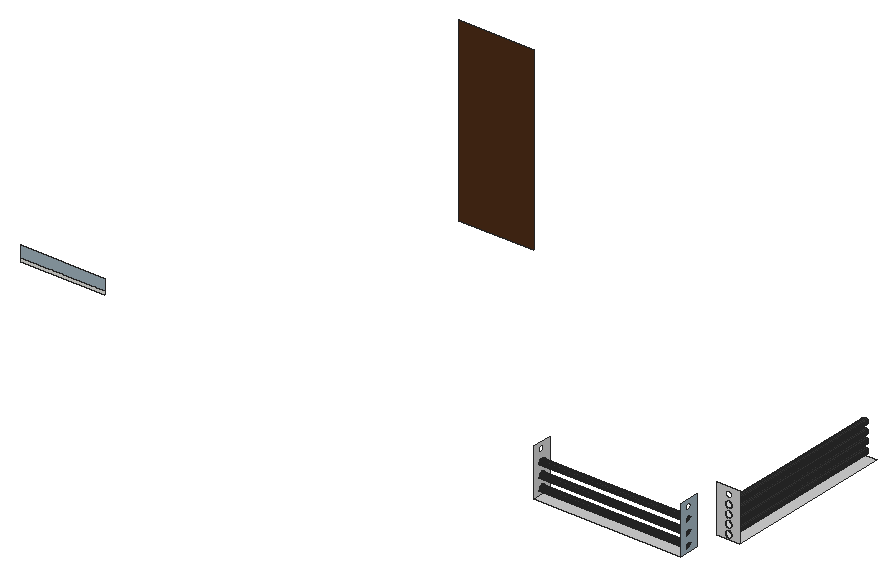
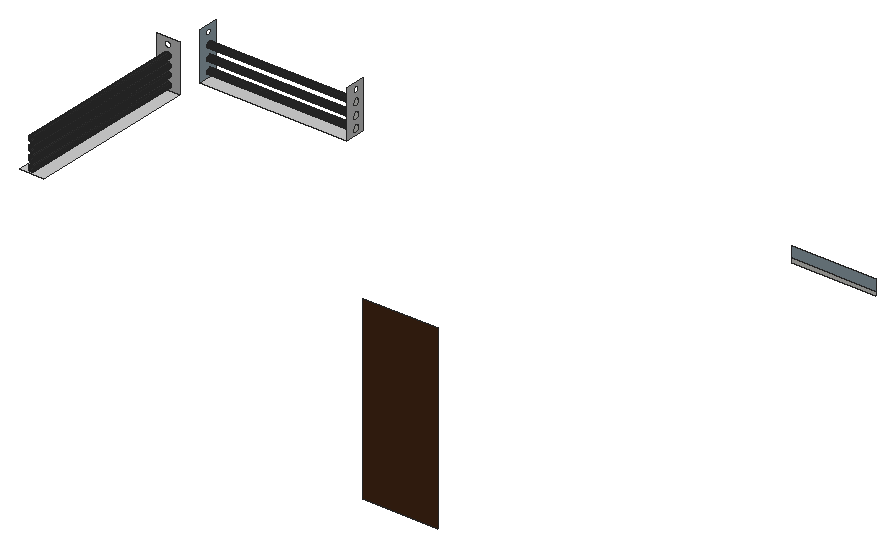
# SketchUp Ruby script. Lengths in inches.
U = 1.inch
M = Sketchup.active_model
def pt(a) = Geom::Point3d.new(a.map { |v| v * U })
def face(e, loops, mat)
  f = e.add_face(loops[0].map { |a| pt(a) })
  loops[1..].each { |l| e.add_face(l.map { |a| pt(a) }).erase! }
  f.material = f.back_material = mat if mat
  f
end
# faces: each face lists its corners as indices into pts; further lists are holes
def faces(e, pts, list, mat = nil) = list.each { |f| face(e, (f[0].is_a?(Array) ? f : [f]).map { |l| l.map { |i| pts[i] } }, mat) }
# xy, xz, yz: faces in a plane at the given z, y or x. An outline is a flat list of corners, or four numbers for a rectangle; further outlines are holes
def ring(l) = l.size == 4 ? [[l[0], l[1]], [l[2], l[1]], [l[2], l[3]], [l[0], l[3]]] : l.each_slice(2).to_a
def flat(e, list, mat, &to3) = list.each { |f| face(e, (f[0].is_a?(Array) ? f : [f]).map { |l| ring(l).map { |u, v| to3.(u, v) } }, mat) }
def xy(e, z, list, mat = nil) = flat(e, list, mat) { |x, y| [x, y, z] }
def xz(e, y, list, mat = nil) = flat(e, list, mat) { |x, z| [x, y, z] }
def yz(e, x, list, mat = nil) = flat(e, list, mat) { |y, z| [x, y, z] }
def lines(e, pts, list) = list.each { |a, b| e.add_line(pt(pts[a]), pt(pts[b])) }
# prism: a flat outline (further loops are holes) pulled along v
def prism(e, loops, v, mat = nil)
  f = face(e, loops, mat); d = Geom::Vector3d.new(v.map { |x| x * U })
  f.pushpull(f.normal.samedirection?(d) ? d.length : -d.length)
end
def box(e, o, s, mat = nil) = prism(e, [[o, [o[0] + s[0], o[1], o[2]], [o[0] + s[0], o[1] + s[1], o[2]], [o[0], o[1] + s[1], o[2]]]], [0, 0, s[2]], mat)
def at(x, y, z, deg = 0) = Geom::Transformation.translation(pt([x, y, z])) * Geom::Transformation.rotation(ORIGIN, Z_AXIS, deg.degrees)
def axes(o, x, y, z) = Geom::Transformation.new([*x, 0, *y, 0, *z, 0, *pt(o).to_a, 1])
def part(name) = M.definitions.add(name)
# library, detail: a bought-in or finely detailed component or shape, given as its bounding box
def library(name, o, s) = part(name).tap { |d| box(d.entities, o, s) }
def detail(e, o, s) = box(e.add_group.entities, o, s)
def put(e, d, t, mat = nil) = e.add_instance(d, t).tap { |i| i.material = mat if mat }
def group(e, t, mat = nil) = e.add_group.tap { |g| g.transformation = t; g.material = mat if mat }.entities
root = M.entities
M.materials.add("[Carrera Marble]").color = [207, 207, 207]
M.materials.add("[Color M07]").color = [58, 58, 58]
M.materials.add("[Formica Speckled Grey]").color = [157, 176, 186]
M.materials.add("[Quartz Light Grey]").color = [251, 251, 252]
M.materials.add("[Wood Veneer 01]").color = [76, 44, 23]
xy(root,72.8125,[[580.71,195.25,736.96,216.53],[736.96,242.62,761.74,423.625]],"[Carrera Marble]")
xz(root,195.25,[[36.42,107.15,126.39,111.12]])
xz(root,195.25,[[36.42,111.12,126.39,122.8125]],"[Formica Speckled Grey]")
xz(root,242.62,[[[736.96,72.8125,761.74,122.8125],[749.95,112.77,749.11,112.88,748.32,113.2,747.65,113.72,747.13,114.39,746.81,115.18,746.7,116.02,746.81,116.86,747.13,117.64,747.65,118.32,748.32,118.83,749.11,119.16,749.95,119.27,750.79,119.16,751.57,118.83,752.24,118.32,752.76,117.64,753.09,116.86,753.2,116.02,753.09,115.18,752.76,114.39,752.24,113.72,751.57,113.2,750.79,112.88],[749.95,74.64,749.11,74.75,748.32,75.08,747.65,75.59,747.13,76.27,746.81,77.05,746.7,77.89,746.81,78.73,747.13,79.52,747.65,80.19,748.32,80.71,749.11,81.03,749.95,81.14,750.79,81.03,751.57,80.71,752.24,80.19,752.76,79.52,753.09,78.73,753.2,77.89,753.09,77.05,752.76,76.27,752.24,75.59,751.57,75.08,750.79,74.75],[749.95,102.77,749.11,102.88,748.32,103.2,747.65,103.72,747.13,104.39,746.81,105.18,746.7,106.02,746.81,106.86,747.13,107.64,747.65,108.32,748.32,108.83,749.11,109.16,749.95,109.27,750.79,109.16,751.57,108.83,752.24,108.32,752.76,107.64,753.09,106.86,753.2,106.02,753.09,105.18,752.76,104.39,752.24,103.72,751.57,103.2,750.79,102.88],[749.95,84.2,749.11,84.32,748.32,84.64,747.65,85.16,747.13,85.83,746.81,86.61,746.7,87.45,746.81,88.3,747.13,89.08,747.65,89.75,748.32,90.27,749.11,90.59,749.95,90.7,750.79,90.59,751.57,90.27,752.24,89.75,752.76,89.08,753.09,88.3,753.2,87.45,753.09,86.61,752.76,85.83,752.24,85.16,751.57,84.64,750.79,84.32],[749.95,93.33,749.11,93.44,748.32,93.77,747.65,94.28,747.13,94.95,746.81,95.74,746.7,96.58,746.81,97.42,747.13,98.2,747.65,98.88,748.32,99.39,749.11,99.72,749.95,99.83,750.79,99.72,751.57,99.39,752.24,98.88,752.76,98.2,753.09,97.42,753.2,96.58,753.09,95.74,752.76,94.95,752.24,94.28,751.57,93.77,750.79,93.44]]],"[Carrera Marble]")
xz(root,242.62,[[749.95,74.64,750.79,74.75,751.57,75.08,752.24,75.59,752.76,76.27,753.09,77.05,753.2,77.89,753.09,78.73,752.76,79.52,752.24,80.19,751.57,80.71,750.79,81.03,749.95,81.14,749.11,81.03,748.32,80.71,747.65,80.19,747.13,79.52,746.81,78.73,746.7,77.89,746.81,77.05,747.13,76.27,747.65,75.59,748.32,75.08,749.11,74.75],[749.95,84.2,750.79,84.32,751.57,84.64,752.24,85.16,752.76,85.83,753.09,86.61,753.2,87.45,753.09,88.3,752.76,89.08,752.24,89.75,751.57,90.27,750.79,90.59,749.95,90.7,749.11,90.59,748.32,90.27,747.65,89.75,747.13,89.08,746.81,88.3,746.7,87.45,746.81,86.61,747.13,85.83,747.65,85.16,748.32,84.64,749.11,84.32],[749.95,93.33,750.79,93.44,751.57,93.77,752.24,94.28,752.76,94.95,753.09,95.74,753.2,96.58,753.09,97.42,752.76,98.2,752.24,98.88,751.57,99.39,750.79,99.72,749.95,99.83,749.11,99.72,748.32,99.39,747.65,98.88,747.13,98.2,746.81,97.42,746.7,96.58,746.81,95.74,747.13,94.95,747.65,94.28,748.32,93.77,749.11,93.44],[749.95,102.77,750.79,102.88,751.57,103.2,752.24,103.72,752.76,104.39,753.09,105.18,753.2,106.02,753.09,106.86,752.76,107.64,752.24,108.32,751.57,108.83,750.79,109.16,749.95,109.27,749.11,109.16,748.32,108.83,747.65,108.32,747.13,107.64,746.81,106.86,746.7,106.02,746.81,105.18,747.13,104.39,747.65,103.72,748.32,103.2,749.11,102.88]],"[Quartz Light Grey]")
xz(root,602.92,[[175.34,16.18,255.42,206.57]],"[Wood Veneer 01]")
yz(root,580.71,[[205.03,76.17,204.24,76.27,203.5,76.58,202.87,77.06,202.38,77.7,202.08,78.4375,201.97,79.23,202.08,80.02,202.38,80.76,202.87,81.4,203.5,81.88,204.24,82.1875,205.03,82.29,205.83,82.1875,206.57,81.88,207.2,81.4,207.6875,80.76,207.99,80.02,208.1,79.23,207.99,78.4375,207.6875,77.7,207.2,77.06,206.57,76.58,205.83,76.27],[205.03,88.54,204.24,88.65,203.5,88.95,202.87,89.44,202.38,90.07,202.08,90.8125,201.97,91.61,202.08,92.4,202.38,93.14,202.87,93.77,203.5,94.26,204.24,94.5625,205.03,94.67,205.83,94.5625,206.57,94.26,207.2,93.77,207.6875,93.14,207.99,92.4,208.1,91.61,207.99,90.8125,207.6875,90.07,207.2,89.44,206.57,88.95,205.83,88.65],[205.03,101.48,204.24,101.58,203.5,101.89,202.87,102.38,202.38,103.01,202.08,103.75,201.97,104.54,202.08,105.34,202.38,106.07,202.87,106.71,203.5,107.2,204.24,107.5,205.03,107.61,205.83,107.5,206.57,107.2,207.2,106.71,207.6875,106.07,207.99,105.34,208.1,104.54,207.99,103.75,207.6875,103.01,207.2,102.38,206.57,101.89,205.83,101.58]])
yz(root,580.71,[[[195.25,72.8125,216.53,122.8125],[205.03,76.17,204.24,76.27,203.5,76.58,202.87,77.06,202.38,77.7,202.08,78.4375,201.97,79.23,202.08,80.02,202.38,80.76,202.87,81.4,203.5,81.88,204.24,82.1875,205.03,82.29,205.83,82.1875,206.57,81.88,207.2,81.4,207.6875,80.76,207.99,80.02,208.1,79.23,207.99,78.4375,207.6875,77.7,207.2,77.06,206.57,76.58,205.83,76.27],[205.03,101.48,204.24,101.58,203.5,101.89,202.87,102.38,202.38,103.01,202.08,103.75,201.97,104.54,202.08,105.34,202.38,106.07,202.87,106.71,203.5,107.2,204.24,107.5,205.03,107.61,205.83,107.5,206.57,107.2,207.2,106.71,207.6875,106.07,207.99,105.34,208.1,104.54,207.99,103.75,207.6875,103.01,207.2,102.38,206.57,101.89,205.83,101.58],[205.03,88.54,204.24,88.65,203.5,88.95,202.87,89.44,202.38,90.07,202.08,90.8125,201.97,91.61,202.08,92.4,202.38,93.14,202.87,93.77,203.5,94.26,204.24,94.5625,205.03,94.67,205.83,94.5625,206.57,94.26,207.2,93.77,207.6875,93.14,207.99,92.4,208.1,91.61,207.99,90.8125,207.6875,90.07,207.2,89.44,206.57,88.95,205.83,88.65],[205.03,113.17,204.24,113.27,203.5,113.58,202.87,114.06,202.38,114.7,202.08,115.4375,201.97,116.23,202.08,117.02,202.38,117.76,202.87,118.4,203.5,118.88,204.24,119.1875,205.03,119.29,205.83,119.1875,206.57,118.88,207.2,118.4,207.6875,117.76,207.99,117.02,208.1,116.23,207.99,115.4375,207.6875,114.7,207.2,114.06,206.57,113.58,205.83,113.27]]],"[Carrera Marble]")
yz(root,736.96,[[[195.25,72.8125,216.53,122.8125],[205.03,113.17,204.24,113.27,203.5,113.58,202.87,114.06,202.38,114.7,202.08,115.4375,201.97,116.23,202.08,117.02,202.38,117.76,202.87,118.4,203.5,118.88,204.24,119.1875,205.03,119.29,205.83,119.1875,206.57,118.88,207.2,118.4,207.6875,117.76,207.99,117.02,208.1,116.23,207.99,115.4375,207.6875,114.7,207.2,114.06,206.57,113.58,205.83,113.27],[205.03,101.48,204.24,101.58,203.5,101.89,202.87,102.38,202.38,103.01,202.08,103.75,201.97,104.54,202.08,105.34,202.38,106.07,202.87,106.71,203.5,107.2,204.24,107.5,205.03,107.61,205.83,107.5,206.57,107.2,207.2,106.71,207.6875,106.07,207.99,105.34,208.1,104.54,207.99,103.75,207.6875,103.01,207.2,102.38,206.57,101.89,205.83,101.58],[205.03,88.54,204.24,88.65,203.5,88.95,202.87,89.44,202.38,90.07,202.08,90.8125,201.97,91.61,202.08,92.4,202.38,93.14,202.87,93.77,203.5,94.26,204.24,94.5625,205.03,94.67,205.83,94.5625,206.57,94.26,207.2,93.77,207.6875,93.14,207.99,92.4,208.1,91.61,207.99,90.8125,207.6875,90.07,207.2,89.44,206.57,88.95,205.83,88.65],[205.03,76.17,204.24,76.27,203.5,76.58,202.87,77.06,202.38,77.7,202.08,78.4375,201.97,79.23,202.08,80.02,202.38,80.76,202.87,81.4,203.5,81.88,204.24,82.1875,205.03,82.29,205.83,82.1875,206.57,81.88,207.2,81.4,207.6875,80.76,207.99,80.02,208.1,79.23,207.99,78.4375,207.6875,77.7,207.2,77.06,206.57,76.58,205.83,76.27]]],"[Formica Speckled Grey]")
p = [[749.95,242.62,74.64],[749.11,242.62,74.75],[749.11,423.625,74.75],[749.95,423.625,74.64],[750.79,242.62,74.75],[750.79,423.625,74.75],
  [748.32,242.62,75.08],[748.32,423.625,75.08],[751.57,242.62,75.08],[751.57,423.625,75.08],[747.65,242.62,75.59],[747.65,423.625,75.59],
  [752.24,242.62,75.59],[752.24,423.625,75.59],[747.13,242.62,76.27],[747.13,423.625,76.27],[752.76,242.62,76.27],[752.76,423.625,76.27],
  [580.71,204.24,76.27],[580.71,205.03,76.17],[736.96,205.03,76.17],[736.96,204.24,76.27],[580.71,205.83,76.27],[736.96,205.83,76.27],
  [580.71,203.5,76.58],[736.96,203.5,76.58],[580.71,206.57,76.58],[736.96,206.57,76.58],[746.81,242.62,77.05],[746.81,423.625,77.05],
  [753.09,242.62,77.05],[753.09,423.625,77.05],[580.71,202.87,77.06],[736.96,202.87,77.06],[580.71,207.2,77.06],[736.96,207.2,77.06],
  [580.71,202.38,77.7],[736.96,202.38,77.7],[580.71,207.6875,77.7],[736.96,207.6875,77.7],[746.7,242.62,77.89],[746.7,423.625,77.89],
  [753.2,242.62,77.89],[753.2,423.625,77.89],[580.71,202.08,78.4375],[736.96,202.08,78.4375],[580.71,207.99,78.4375],[736.96,207.99,78.4375],
  [746.81,242.62,78.73],[746.81,423.625,78.73],[753.09,242.62,78.73],[753.09,423.625,78.73],[580.71,201.97,79.23],[736.96,201.97,79.23],
  [580.71,208.1,79.23],[736.96,208.1,79.23],[747.13,242.62,79.52],[747.13,423.625,79.52],[752.76,242.62,79.52],[752.76,423.625,79.52],
  [580.71,202.08,80.02],[736.96,202.08,80.02],[580.71,207.99,80.02],[736.96,207.99,80.02],[747.65,242.62,80.19],[747.65,423.625,80.19],
  [752.24,242.62,80.19],[752.24,423.625,80.19],[580.71,202.38,80.76],[736.96,202.38,80.76],[580.71,207.6875,80.76],[736.96,207.6875,80.76],
  [748.32,242.62,80.71],[748.32,423.625,80.71],[751.57,242.62,80.71],[751.57,423.625,80.71],[749.11,242.62,81.03],[749.11,423.625,81.03],
  [750.79,242.62,81.03],[750.79,423.625,81.03],[580.71,202.87,81.4],[736.96,202.87,81.4],[580.71,207.2,81.4],[736.96,207.2,81.4],
  [749.95,242.62,81.14],[749.95,423.625,81.14],[580.71,203.5,81.88],[736.96,203.5,81.88],[580.71,206.57,81.88],[736.96,206.57,81.88],
  [580.71,204.24,82.1875],[736.96,204.24,82.1875],[580.71,205.83,82.1875],[736.96,205.83,82.1875],[580.71,205.03,82.29],[736.96,205.03,82.29],
  [749.95,242.62,84.2],[749.11,242.62,84.32],[749.11,423.625,84.32],[749.95,423.625,84.2],[750.79,242.62,84.32],[750.79,423.625,84.32],
  [748.32,242.62,84.64],[748.32,423.625,84.64],[751.57,242.62,84.64],[751.57,423.625,84.64],[747.65,242.62,85.16],[747.65,423.625,85.16],
  [752.24,242.62,85.16],[752.24,423.625,85.16],[747.13,242.62,85.83],[747.13,423.625,85.83],[752.76,242.62,85.83],[752.76,423.625,85.83],
  [746.81,242.62,86.61],[746.81,423.625,86.61],[753.09,242.62,86.61],[753.09,423.625,86.61],[746.7,242.62,87.45],[746.7,423.625,87.45],
  [753.2,242.62,87.45],[753.2,423.625,87.45],[746.81,242.62,88.3],[746.81,423.625,88.3],[753.09,242.62,88.3],[753.09,423.625,88.3],
  [747.13,242.62,89.08],[747.13,423.625,89.08],[752.76,242.62,89.08],[752.76,423.625,89.08],[580.71,204.24,88.65],[580.71,205.03,88.54],
  [736.96,205.03,88.54],[736.96,204.24,88.65],[580.71,205.83,88.65],[736.96,205.83,88.65],[580.71,203.5,88.95],[736.96,203.5,88.95],
  [580.71,206.57,88.95],[736.96,206.57,88.95],[580.71,202.87,89.44],[736.96,202.87,89.44],[580.71,207.2,89.44],[736.96,207.2,89.44],
  [747.65,242.62,89.75],[747.65,423.625,89.75],[752.24,242.62,89.75],[752.24,423.625,89.75],[580.71,202.38,90.07],[736.96,202.38,90.07],
  [580.71,207.6875,90.07],[736.96,207.6875,90.07],[748.32,242.62,90.27],[748.32,423.625,90.27],[751.57,242.62,90.27],[751.57,423.625,90.27],
  [580.71,202.08,90.8125],[736.96,202.08,90.8125],[580.71,207.99,90.8125],[736.96,207.99,90.8125],[749.11,242.62,90.59],[749.11,423.625,90.59],
  [750.79,242.62,90.59],[750.79,423.625,90.59],[749.95,242.62,90.7],[749.95,423.625,90.7],[580.71,201.97,91.61],[736.96,201.97,91.61],
  [580.71,208.1,91.61],[736.96,208.1,91.61],[580.71,202.08,92.4],[736.96,202.08,92.4],[580.71,207.99,92.4],[736.96,207.99,92.4],
  [580.71,202.38,93.14],[736.96,202.38,93.14],[580.71,207.6875,93.14],[736.96,207.6875,93.14],[580.71,202.87,93.77],[736.96,202.87,93.77],
  [580.71,207.2,93.77],[736.96,207.2,93.77],[749.95,242.62,93.33],[749.11,242.62,93.44],[749.11,423.625,93.44],[749.95,423.625,93.33],
  [750.79,242.62,93.44],[750.79,423.625,93.44],[748.32,242.62,93.77],[748.32,423.625,93.77],[751.57,242.62,93.77],[751.57,423.625,93.77],
  [580.71,203.5,94.26],[736.96,203.5,94.26],[580.71,206.57,94.26],[736.96,206.57,94.26],[747.65,242.62,94.28],[747.65,423.625,94.28],
  [752.24,242.62,94.28],[752.24,423.625,94.28],[580.71,204.24,94.5625],[736.96,204.24,94.5625],[580.71,205.83,94.5625],[736.96,205.83,94.5625],
  [747.13,242.62,94.95],[747.13,423.625,94.95],[752.76,242.62,94.95],[752.76,423.625,94.95],[580.71,205.03,94.67],[736.96,205.03,94.67],
  [746.81,242.62,95.74],[746.81,423.625,95.74],[753.09,242.62,95.74],[753.09,423.625,95.74],[746.7,242.62,96.58],[746.7,423.625,96.58],
  [753.2,242.62,96.58],[753.2,423.625,96.58],[746.81,242.62,97.42],[746.81,423.625,97.42],[753.09,242.62,97.42],[753.09,423.625,97.42],
  [747.13,242.62,98.2],[747.13,423.625,98.2],[752.76,242.62,98.2],[752.76,423.625,98.2],[747.65,242.62,98.88],[747.65,423.625,98.88],
  [752.24,242.62,98.88],[752.24,423.625,98.88],[748.32,242.62,99.39],[748.32,423.625,99.39],[751.57,242.62,99.39],[751.57,423.625,99.39],
  [749.11,242.62,99.72],[749.11,423.625,99.72],[750.79,242.62,99.72],[750.79,423.625,99.72],[749.95,242.62,99.83],[749.95,423.625,99.83],
  [580.71,204.24,101.58],[580.71,205.03,101.48],[736.96,205.03,101.48],[736.96,204.24,101.58],[580.71,205.83,101.58],[736.96,205.83,101.58],
  [580.71,203.5,101.89],[736.96,203.5,101.89],[580.71,206.57,101.89],[736.96,206.57,101.89],[580.71,202.87,102.38],[736.96,202.87,102.38],
  [580.71,207.2,102.38],[736.96,207.2,102.38],[580.71,202.38,103.01],[736.96,202.38,103.01],[580.71,207.6875,103.01],[736.96,207.6875,103.01],
  [749.95,242.62,102.77],[749.11,242.62,102.88],[749.11,423.625,102.88],[749.95,423.625,102.77],[750.79,242.62,102.88],[750.79,423.625,102.88],
  [748.32,242.62,103.2],[748.32,423.625,103.2],[751.57,242.62,103.2],[751.57,423.625,103.2],[580.71,202.08,103.75],[736.96,202.08,103.75],
  [580.71,207.99,103.75],[736.96,207.99,103.75],[747.65,242.62,103.72],[747.65,423.625,103.72],[752.24,242.62,103.72],[752.24,423.625,103.72],
  [747.13,242.62,104.39],[747.13,423.625,104.39],[752.76,242.62,104.39],[752.76,423.625,104.39],[580.71,201.97,104.54],[736.96,201.97,104.54],
  [580.71,208.1,104.54],[736.96,208.1,104.54],[746.81,242.62,105.18],[746.81,423.625,105.18],[753.09,242.62,105.18],[753.09,423.625,105.18],
  [580.71,202.08,105.34],[736.96,202.08,105.34],[580.71,207.99,105.34],[736.96,207.99,105.34],[746.7,242.62,106.02],[746.7,423.625,106.02],
  [753.2,242.62,106.02],[753.2,423.625,106.02],[580.71,202.38,106.07],[736.96,202.38,106.07],[580.71,207.6875,106.07],[736.96,207.6875,106.07],
  [746.81,242.62,106.86],[746.81,423.625,106.86],[753.09,242.62,106.86],[753.09,423.625,106.86],[580.71,202.87,106.71],[736.96,202.87,106.71],
  [580.71,207.2,106.71],[736.96,207.2,106.71],[580.71,203.5,107.2],[736.96,203.5,107.2],[580.71,206.57,107.2],[736.96,206.57,107.2],
  [747.13,242.62,107.64],[747.13,423.625,107.64],[752.76,242.62,107.64],[752.76,423.625,107.64],[580.71,204.24,107.5],[736.96,204.24,107.5],
  [580.71,205.83,107.5],[736.96,205.83,107.5],[580.71,205.03,107.61],[736.96,205.03,107.61],[747.65,242.62,108.32],[747.65,423.625,108.32],
  [752.24,242.62,108.32],[752.24,423.625,108.32],[748.32,242.62,108.83],[748.32,423.625,108.83],[751.57,242.62,108.83],[751.57,423.625,108.83],
  [749.11,242.62,109.16],[749.11,423.625,109.16],[750.79,242.62,109.16],[750.79,423.625,109.16],[749.95,242.62,109.27],[749.95,423.625,109.27]]
faces(root,p,[[0,1,2,3],[4,0,3,5],[1,6,7,2],[8,4,5,9],[6,10,11,7],[12,8,9,13],[10,14,15,11],[16,12,13,17],
  [18,19,20,21],[19,22,23,20],[24,18,21,25],[22,26,27,23],[14,28,29,15],[30,16,17,31],[32,24,25,33],[26,34,35,27],
  [36,32,33,37],[34,38,39,35],[28,40,41,29],[42,30,31,43],[44,36,37,45],[38,46,47,39],[40,48,49,41],[50,42,43,51],
  [52,44,45,53],[46,54,55,47],[48,56,57,49],[58,50,51,59],[60,52,53,61],[54,62,63,55],[56,64,65,57],[66,58,59,67],
  [68,60,61,69],[62,70,71,63],[64,72,73,65],[74,66,67,75],[72,76,77,73],[78,74,75,79],[80,68,69,81],[70,82,83,71],
  [76,84,85,77],[84,78,79,85],[86,80,81,87],[82,88,89,83],[90,86,87,91],[88,92,93,89],[94,90,91,95],[92,94,95,93],
  [96,97,98,99],[100,96,99,101],[97,102,103,98],[104,100,101,105],[102,106,107,103],[108,104,105,109],[106,110,111,107],[112,108,109,113],
  [110,114,115,111],[116,112,113,117],[114,118,119,115],[120,116,117,121],[118,122,123,119],[124,120,121,125],[122,126,127,123],[128,124,125,129],
  [130,131,132,133],[131,134,135,132],[136,130,133,137],[134,138,139,135],[140,136,137,141],[138,142,143,139],[126,144,145,127],[146,128,129,147],
  [148,140,141,149],[142,150,151,143],[144,152,153,145],[154,146,147,155],[156,148,149,157],[150,158,159,151],[152,160,161,153],[162,154,155,163],
  [160,164,165,161],[164,162,163,165],[166,156,157,167],[158,168,169,159],[170,166,167,171],[168,172,173,169],[174,170,171,175],[172,176,177,173],
  [178,174,175,179],[176,180,181,177],[182,183,184,185],[186,182,185,187],[183,188,189,184],[190,186,187,191],[192,178,179,193],[180,194,195,181],
  [188,196,197,189],[198,190,191,199],[200,192,193,201],[194,202,203,195],[196,204,205,197],[206,198,199,207],[208,200,201,209],[202,208,209,203],
  [204,210,211,205],[212,206,207,213],[210,214,215,211],[216,212,213,217],[214,218,219,215],[220,216,217,221],[218,222,223,219],[224,220,221,225],
  [222,226,227,223],[228,224,225,229],[226,230,231,227],[232,228,229,233],[230,234,235,231],[236,232,233,237],[234,238,239,235],[238,236,237,239],
  [240,241,242,243],[241,244,245,242],[246,240,243,247],[244,248,249,245],[250,246,247,251],[248,252,253,249],[254,250,251,255],[252,256,257,253],
  [258,259,260,261],[262,258,261,263],[259,264,265,260],[266,262,263,267],[268,254,255,269],[256,270,271,257],[264,272,273,265],[274,266,267,275],
  [272,276,277,273],[278,274,275,279],[280,268,269,281],[270,282,283,271],[276,284,285,277],[286,278,279,287],[288,280,281,289],[282,290,291,283],
  [284,292,293,285],[294,286,287,295],[296,288,289,297],[290,298,299,291],[292,300,301,293],[302,294,295,303],[304,296,297,305],[298,306,307,299],
  [308,304,305,309],[306,310,311,307],[300,312,313,301],[314,302,303,315],[316,308,309,317],[310,318,319,311],[320,316,317,321],[318,320,321,319],
  [312,322,323,313],[324,314,315,325],[322,326,327,323],[328,324,325,329],[326,330,331,327],[332,328,329,333],[330,334,335,331],[334,332,333,335]],"[Color M07]")
